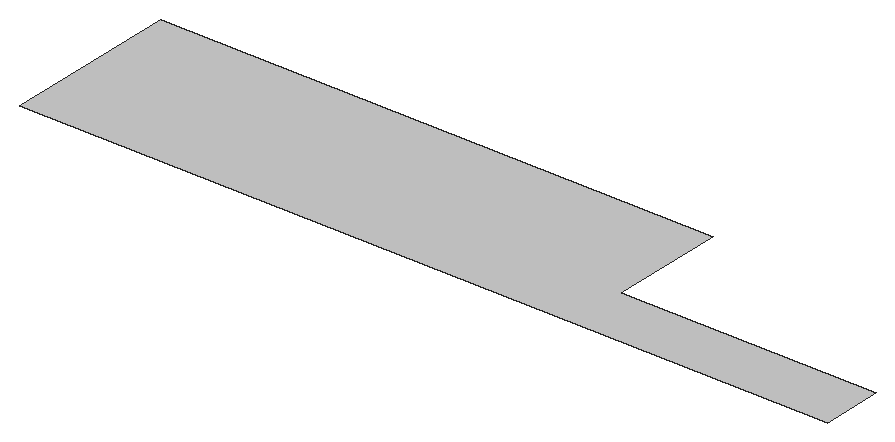
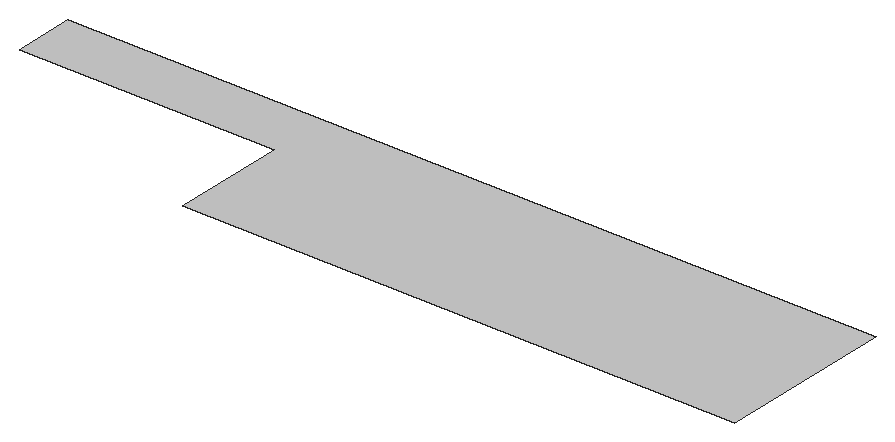
# SketchUp Ruby script. Lengths in inches.
U = 1.inch
M = Sketchup.active_model
def pt(a) = Geom::Point3d.new(a.map { |v| v * U })
def face(e, loops, mat)
  f = e.add_face(loops[0].map { |a| pt(a) })
  loops[1..].each { |l| e.add_face(l.map { |a| pt(a) }).erase! }
  f.material = f.back_material = mat if mat
  f
end
# faces: each face lists its corners as indices into pts; further lists are holes
def faces(e, pts, list, mat = nil) = list.each { |f| face(e, (f[0].is_a?(Array) ? f : [f]).map { |l| l.map { |i| pts[i] } }, mat) }
# xy, xz, yz: faces in a plane at the given z, y or x. An outline is a flat list of corners, or four numbers for a rectangle; further outlines are holes
def ring(l) = l.size == 4 ? [[l[0], l[1]], [l[2], l[1]], [l[2], l[3]], [l[0], l[3]]] : l.each_slice(2).to_a
def flat(e, list, mat, &to3) = list.each { |f| face(e, (f[0].is_a?(Array) ? f : [f]).map { |l| ring(l).map { |u, v| to3.(u, v) } }, mat) }
def xy(e, z, list, mat = nil) = flat(e, list, mat) { |x, y| [x, y, z] }
def xz(e, y, list, mat = nil) = flat(e, list, mat) { |x, z| [x, y, z] }
def yz(e, x, list, mat = nil) = flat(e, list, mat) { |y, z| [x, y, z] }
def lines(e, pts, list) = list.each { |a, b| e.add_line(pt(pts[a]), pt(pts[b])) }
# prism: a flat outline (further loops are holes) pulled along v
def prism(e, loops, v, mat = nil)
  f = face(e, loops, mat); d = Geom::Vector3d.new(v.map { |x| x * U })
  f.pushpull(f.normal.samedirection?(d) ? d.length : -d.length)
end
def box(e, o, s, mat = nil) = prism(e, [[o, [o[0] + s[0], o[1], o[2]], [o[0] + s[0], o[1] + s[1], o[2]], [o[0], o[1] + s[1], o[2]]]], [0, 0, s[2]], mat)
def at(x, y, z, deg = 0) = Geom::Transformation.translation(pt([x, y, z])) * Geom::Transformation.rotation(ORIGIN, Z_AXIS, deg.degrees)
def axes(o, x, y, z) = Geom::Transformation.new([*x, 0, *y, 0, *z, 0, *pt(o).to_a, 1])
def part(name) = M.definitions.add(name)
# library, detail: a bought-in or finely detailed component or shape, given as its bounding box
def library(name, o, s) = part(name).tap { |d| box(d.entities, o, s) }
def detail(e, o, s) = box(e.add_group.entities, o, s)
def put(e, d, t, mat = nil) = e.add_instance(d, t).tap { |i| i.material = mat if mat }
def group(e, t, mat = nil) = e.add_group.tap { |g| g.transformation = t; g.material = mat if mat }.entities
root = M.entities
M.materials.add("[Carrera Marble]").color = [207, 207, 207]
xy(root,0,[[0,81.92,0,184.11,321.5,184.11,321.5,117.03,469.67,117.03,469.67,81.92]],"[Carrera Marble]")
